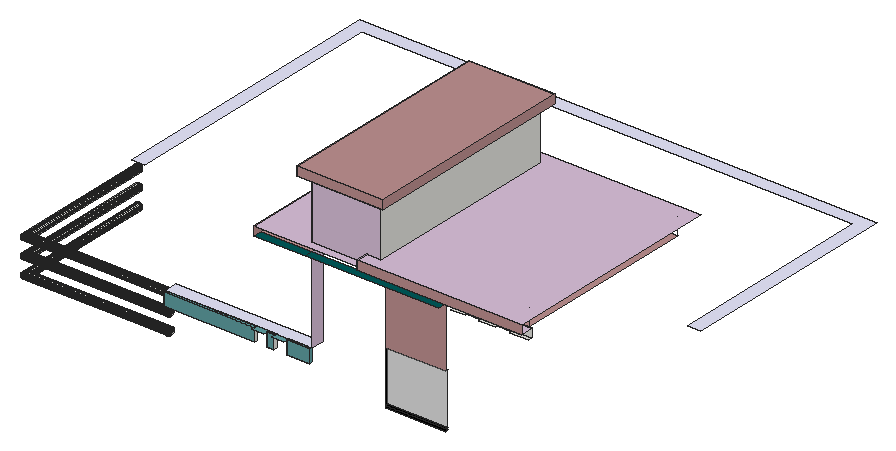
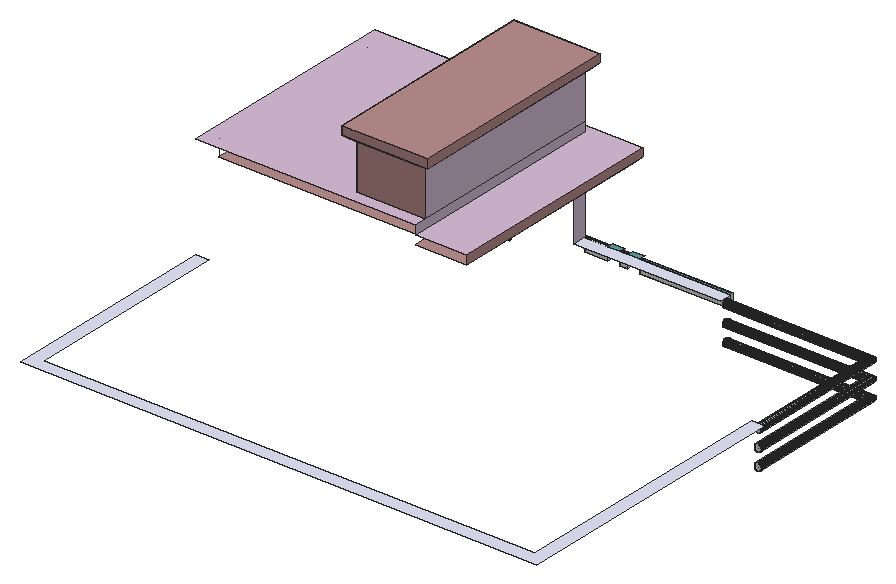
# SketchUp Ruby script. Lengths in inches.
U = 1.inch
M = Sketchup.active_model
def pt(a) = Geom::Point3d.new(a.map { |v| v * U })
def face(e, loops, mat)
  f = e.add_face(loops[0].map { |a| pt(a) })
  loops[1..].each { |l| e.add_face(l.map { |a| pt(a) }).erase! }
  f.material = f.back_material = mat if mat
  f
end
# faces: each face lists its corners as indices into pts; further lists are holes
def faces(e, pts, list, mat = nil) = list.each { |f| face(e, (f[0].is_a?(Array) ? f : [f]).map { |l| l.map { |i| pts[i] } }, mat) }
# xy, xz, yz: faces in a plane at the given z, y or x. An outline is a flat list of corners, or four numbers for a rectangle; further outlines are holes
def ring(l) = l.size == 4 ? [[l[0], l[1]], [l[2], l[1]], [l[2], l[3]], [l[0], l[3]]] : l.each_slice(2).to_a
def flat(e, list, mat, &to3) = list.each { |f| face(e, (f[0].is_a?(Array) ? f : [f]).map { |l| ring(l).map { |u, v| to3.(u, v) } }, mat) }
def xy(e, z, list, mat = nil) = flat(e, list, mat) { |x, y| [x, y, z] }
def xz(e, y, list, mat = nil) = flat(e, list, mat) { |x, z| [x, y, z] }
def yz(e, x, list, mat = nil) = flat(e, list, mat) { |y, z| [x, y, z] }
def lines(e, pts, list) = list.each { |a, b| e.add_line(pt(pts[a]), pt(pts[b])) }
# prism: a flat outline (further loops are holes) pulled along v
def prism(e, loops, v, mat = nil)
  f = face(e, loops, mat); d = Geom::Vector3d.new(v.map { |x| x * U })
  f.pushpull(f.normal.samedirection?(d) ? d.length : -d.length)
end
def box(e, o, s, mat = nil) = prism(e, [[o, [o[0] + s[0], o[1], o[2]], [o[0] + s[0], o[1] + s[1], o[2]], [o[0], o[1] + s[1], o[2]]]], [0, 0, s[2]], mat)
def at(x, y, z, deg = 0) = Geom::Transformation.translation(pt([x, y, z])) * Geom::Transformation.rotation(ORIGIN, Z_AXIS, deg.degrees)
def axes(o, x, y, z) = Geom::Transformation.new([*x, 0, *y, 0, *z, 0, *pt(o).to_a, 1])
def part(name) = M.definitions.add(name)
# library, detail: a bought-in or finely detailed component or shape, given as its bounding box
def library(name, o, s) = part(name).tap { |d| box(d.entities, o, s) }
def detail(e, o, s) = box(e.add_group.entities, o, s)
def put(e, d, t, mat = nil) = e.add_instance(d, t).tap { |i| i.material = mat if mat }
def group(e, t, mat = nil) = e.add_group.tap { |g| g.transformation = t; g.material = mat if mat }.entities
root = M.entities
M.materials.add("[0080_DarkCyan]").color = [0, 89, 89]
M.materials.add("[0081_CadetBlue]").color = [95, 158, 160]
M.materials.add("[0116_Lavender]").color = [230, 230, 250]
M.materials.add("[0118_Thistle]").color = [216, 191, 216]
M.materials.add("[0119_RosyBrown]").color = [188, 143, 143]
M.materials.add("[0137_Black]").color = [0, 0, 0]
M.materials.add("[Translucent Glass Gray]").color = [128, 128, 128]
M.materials["[Translucent Glass Gray]"].alpha = 0.5
xy(root,429,[[528,18,612,21]],"[0137_Black]")
xy(root,432,[[528,18,612,21]],"[0137_Black]")
xy(root,450,[[222,14,348.57,18],[365.51,14,376.32,18],[393.26,14,426,18]],"[0081_CadetBlue]")
xy(root,468,[[348.57,10,365.51,18],[376.32,10,393.26,18],[222,14,348.57,18],[365.51,14,376.32,18],[393.26,14,426,18]],"[0081_CadetBlue]")
xy(root,468,[[222,18,426,36],[12,222,30,222,30,600,714,600,714,312,732,312,732,618,12,618]],"[0116_Lavender]")
xy(root,504,[[528,18,612,21]],"[0137_Black]")
xy(root,588,[[624,12,644.09,12,644.09,15,663.05,15,663.05,12,687.09,12,687.09,15,706.05,15,706.05,12,732,12,732,18,624,18],[389.27,45.6875,387.74,46.01,386.34,46.72,385.18,47.76,384.32,49.07,383.84,50.5625,383.75,52.13,384.07,53.66,384.78,55.06,385.83,56.22,387.14,57.08,388.63,57.57,390.19,57.65,391.72,57.33,393.12,56.62,394.29,55.57,395.14,54.26,395.63,52.77,395.72,51.21,395.39,49.68,394.68,48.28,393.64,47.11,392.33,46.26,390.84,45.77],[389.27,83.6875,387.74,84.01,386.34,84.72,385.18,85.76,384.32,87.07,383.84,88.5625,383.75,90.13,384.07,91.66,384.78,93.06,385.83,94.22,387.14,95.08,388.63,95.57,390.19,95.65,391.72,95.33,393.12,94.62,394.29,93.57,395.14,92.26,395.63,90.77,395.72,89.21,395.39,87.68,394.68,86.28,393.64,85.11,392.33,84.26,390.84,83.77],[389.27,135.125,387.74,135.45,386.34,136.15,385.18,137.2,384.32,138.51,383.84,140,383.75,141.57,384.07,143.1,384.78,144.49,385.83,145.66,387.14,146.52,388.63,147,390.19,147.09,391.72,146.77,393.12,146.06,394.29,145.01,395.14,143.7,395.63,142.21,395.72,140.65,395.39,139.12,394.68,137.72,393.64,136.55,392.33,135.7,390.84,135.21]])
xy(root,588,[[354,6,426,18],[426,6,612,18]],"[0080_DarkCyan]")
xy(root,588,[[[354,18,354,312,426,312,426,294,714,294,714,36,426,36,426,18],[389.27,83.6875,390.84,83.77,392.33,84.26,393.64,85.11,394.68,86.28,395.39,87.68,395.72,89.21,395.63,90.77,395.14,92.26,394.29,93.57,393.12,94.62,391.72,95.33,390.19,95.65,388.63,95.57,387.14,95.08,385.83,94.22,384.78,93.06,384.07,91.66,383.75,90.13,383.84,88.5625,384.32,87.07,385.18,85.76,386.34,84.72,387.74,84.01],[389.27,135.125,390.84,135.21,392.33,135.7,393.64,136.55,394.68,137.72,395.39,139.12,395.72,140.65,395.63,142.21,395.14,143.7,394.29,145.01,393.12,146.06,391.72,146.77,390.19,147.09,388.63,147,387.14,146.52,385.83,145.66,384.78,144.49,384.07,143.1,383.75,141.57,383.84,140,384.32,138.51,385.18,137.2,386.34,136.15,387.74,135.45],[389.27,45.6875,390.84,45.77,392.33,46.26,393.64,47.11,394.68,48.28,395.39,49.68,395.72,51.21,395.63,52.77,395.14,54.26,394.29,55.57,393.12,56.62,391.72,57.33,390.19,57.65,388.63,57.57,387.14,57.08,385.83,56.22,384.78,55.06,384.07,53.66,383.75,52.13,383.84,50.5625,384.32,49.07,385.18,47.76,386.34,46.72,387.74,46.01]]],"[0119_RosyBrown]")
xy(root,600,[[502.63,6,624,18]])
xy(root,600,[[502.63,0,502.63,6,624,6,624,18,732,18,732,0],[354,6,502.63,6,502.63,18,426,18,426,312,354,312]],"[0118_Thistle]")
xy(root,612,[[502.63,0,732,0,732,312,426,312,426,294,522,294,522,18,502.63,18]],"[0118_Thistle]")
xy(root,684,[[426,18,522,294],[426,294,522,306]])
xy(root,684,[[414,6,534,18],[414,18,426,306],[522,18,534,306]],"[0119_RosyBrown]")
xy(root,696,[[414,6,534,306]],"[0119_RosyBrown]")
xz(root,0,[[502.63,600,732,612]],"[0119_RosyBrown]")
xz(root,6,[[414,684,534,696]],"[0119_RosyBrown]")
xz(root,14,[[222,450,348.57,468],[365.51,450,376.32,468],[393.26,450,426,468]],"[0081_CadetBlue]")
xz(root,18,[[222,450,348.57,468],[365.51,450,376.32,468],[393.26,450,426,468],[624,588,732,600]])
xz(root,18,[[426,600,502.63,600,502.63,612,522,612,522,684,426,684]],"[0118_Thistle]")
xz(root,18,[[528,504,612,588]],"[0119_RosyBrown]")
xz(root,18,[[528,429,612,432]],"[0137_Black]")
xz(root,21,[[528,432,612,504]],"[Translucent Glass Gray]")
xz(root,222,[[21.12,407.86,20.59,407.87,20.08,407.94,19.57,408.07,19.07,408.24,18.6,408.47,18.16,408.74,17.74,409.0625,17.36,409.42,17.02,409.82,16.73,410.25,16.48,410.72,16.28,411.2,16.13,411.7,16.04,412.22,16,412.74,16.02,413.26,16.09,413.78,16.21,414.29,16.39,414.78,16.61,415.25,16.89,415.7,17.21,416.11,17.57,416.49,17.97,416.83,18.4,417.125,18.86,417.375,19.34,417.57,19.85,417.72,20.36,417.8125,20.88,417.85,21.41,417.84,21.92,417.77,22.43,417.65,22.93,417.47,23.4,417.24,23.84,416.97,24.26,416.65,24.64,416.29,24.98,415.89,25.27,415.46,25.52,415,25.72,414.51,25.87,414.01,25.96,413.49,26,412.97,25.98,412.45,25.91,411.93,25.79,411.42,25.61,410.93,25.39,410.46,25.11,410.01,24.79,409.6,24.43,409.22,24.03,408.88,23.6,408.58,23.14,408.34,22.66,408.14,22.15,407.99,21.64,407.9],[21.12,431.86,20.59,431.87,20.08,431.94,19.57,432.07,19.07,432.24,18.6,432.47,18.16,432.74,17.74,433.0625,17.36,433.42,17.02,433.82,16.73,434.25,16.48,434.72,16.28,435.2,16.13,435.7,16.04,436.22,16,436.74,16.02,437.26,16.09,437.78,16.21,438.29,16.39,438.78,16.61,439.25,16.89,439.7,17.21,440.11,17.57,440.49,17.97,440.83,18.4,441.125,18.86,441.375,19.34,441.57,19.85,441.72,20.36,441.8125,20.88,441.85,21.41,441.84,21.92,441.77,22.43,441.65,22.93,441.47,23.4,441.24,23.84,440.97,24.26,440.65,24.64,440.29,24.98,439.89,25.27,439.46,25.52,439,25.72,438.51,25.87,438.01,25.96,437.49,26,436.97,25.98,436.45,25.91,435.93,25.79,435.42,25.61,434.93,25.39,434.46,25.11,434.01,24.79,433.6,24.43,433.22,24.03,432.88,23.6,432.58,23.14,432.34,22.66,432.14,22.15,431.99,21.64,431.9],[21.12,455.86,20.59,455.87,20.08,455.94,19.57,456.07,19.07,456.24,18.6,456.47,18.16,456.74,17.74,457.0625,17.36,457.42,17.02,457.82,16.73,458.25,16.48,458.72,16.28,459.2,16.13,459.7,16.04,460.22,16,460.74,16.02,461.26,16.09,461.78,16.21,462.29,16.39,462.78,16.61,463.25,16.89,463.7,17.21,464.11,17.57,464.49,17.97,464.83,18.4,465.125,18.86,465.375,19.34,465.57,19.85,465.72,20.36,465.8125,20.88,465.85,21.41,465.84,21.92,465.77,22.43,465.65,22.93,465.47,23.4,465.24,23.84,464.97,24.26,464.65,24.64,464.29,24.98,463.89,25.27,463.46,25.52,463,25.72,462.51,25.87,462.01,25.96,461.49,26,460.97,25.98,460.45,25.91,459.93,25.79,459.42,25.61,458.93,25.39,458.46,25.11,458.01,24.79,457.6,24.43,457.22,24.03,456.88,23.6,456.58,23.14,456.34,22.66,456.14,22.15,455.99,21.64,455.9]])
xz(root,294,[[426,612,522,684]],"[0119_RosyBrown]")
xz(root,306,[[414,684,534,696]],"[0119_RosyBrown]")
yz(root,222,[[26.48,407.86,25.96,407.95,25.45,408.08,24.97,408.27,24.5,408.51,24.0625,408.79,23.65,409.12,23.28,409.49,22.95,409.9,22.67,410.34,22.43,410.8,22.24,411.29,22.13,411.7,22.11,411.8,22.05,412.14,22.13,411.7,22.28,411.2,22.48,410.72,22.73,410.25,23.02,409.82,23.36,409.42,23.74,409.0625,24.16,408.74,24.6,408.47,25.07,408.24,25.57,408.07,26.08,407.94,26.59,407.87,27.08,407.86],[27.14,407.86,27.64,407.9,28.15,407.99,28.66,408.14,29.14,408.34,29.6,408.58,30.03,408.88,30.43,409.22,30.79,409.6,31.11,410.01,31.39,410.46,31.61,410.93,31.79,411.42,31.91,411.91,31.89,411.8,31.79,411.42,31.76,411.29,31.57,410.8,31.33,410.34,31.05,409.9,30.72,409.49,30.35,409.12,29.9375,408.79,29.5,408.51,29.03,408.27,28.55,408.08,28.04,407.95,27.52,407.86],[31.92,412,31.98,412.4,31.97,412.3125],[22.04,412.24,22.03,412.3125,22.01,412.58],[31.99,412.61,32,412.9,32,412.84],
  [22,412.78,22,412.84,22.01,413.02],[31.98,413.22,31.97,413.4,31.97,413.36],[22.03,413.33,22.03,413.36,22.04,413.45],[31.9,413.82,31.89,413.89,31.89,413.875],[26.48,431.86,25.96,431.95,25.45,432.08,24.97,432.27,24.5,432.51,24.0625,432.79,23.65,433.12,23.28,433.49,22.95,433.9,22.67,434.34,22.43,434.8,22.24,435.29,22.13,435.7,22.11,435.8,22.05,436.14,22.13,435.7,22.28,435.2,22.48,434.72,22.73,434.25,23.02,433.82,23.36,433.42,23.74,433.0625,24.16,432.74,24.6,432.47,25.07,432.24,25.57,432.07,26.08,431.94,26.59,431.87,27.08,431.86],
  [27.14,431.86,27.64,431.9,28.15,431.99,28.66,432.14,29.14,432.34,29.6,432.58,30.03,432.88,30.43,433.22,30.79,433.6,31.11,434.01,31.39,434.46,31.61,434.93,31.79,435.42,31.91,435.91,31.89,435.8,31.79,435.42,31.76,435.29,31.57,434.8,31.33,434.34,31.05,433.9,30.72,433.49,30.35,433.12,29.9375,432.79,29.5,432.51,29.03,432.27,28.55,432.08,28.04,431.95,27.52,431.86],[31.92,436,31.98,436.4,31.97,436.3125],[22.04,436.24,22.03,436.3125,22.01,436.58],[31.99,436.61,32,436.9,32,436.84],[22,436.78,22,436.84,22.01,437.02],
  [31.98,437.22,31.97,437.4,31.97,437.36],[22.03,437.33,22.03,437.36,22.04,437.45],[31.9,437.82,31.89,437.89,31.89,437.875],[14,450,18,468],[26.48,455.86,25.96,455.95,25.45,456.08,24.97,456.27,24.5,456.51,24.0625,456.79,23.65,457.12,23.28,457.49,22.95,457.9,22.67,458.34,22.43,458.8,22.24,459.29,22.13,459.7,22.11,459.8,22.05,460.14,22.13,459.7,22.28,459.2,22.48,458.72,22.73,458.25,23.02,457.82,23.36,457.42,23.74,457.0625,24.16,456.74,24.6,456.47,25.07,456.24,25.57,456.07,26.08,455.94,26.59,455.87,27.08,455.86],
  [27.14,455.86,27.64,455.9,28.15,455.99,28.66,456.14,29.14,456.34,29.6,456.58,30.03,456.88,30.43,457.22,30.79,457.6,31.11,458.01,31.39,458.46,31.61,458.93,31.79,459.42,31.91,459.91,31.89,459.8,31.79,459.42,31.76,459.29,31.57,458.8,31.33,458.34,31.05,457.9,30.72,457.49,30.35,457.12,29.9375,456.79,29.5,456.51,29.03,456.27,28.55,456.08,28.04,455.95,27.52,455.86],[31.92,460,31.98,460.4,31.97,460.3125],[22.04,460.24,22.03,460.3125,22.01,460.58],[31.99,460.61,32,460.9,32,460.84],[22,460.78,22,460.84,22.01,461.02],
  [31.98,461.22,31.97,461.4,31.97,461.36],[22.03,461.33,22.03,461.36,22.04,461.45],[31.9,461.82,31.89,461.89,31.89,461.875]])
yz(root,348.57,[[14,450,18,468]])
yz(root,354,[[6,588,312,600]],"[0119_RosyBrown]")
yz(root,365.51,[[14,450,18,468]])
yz(root,376.32,[[14,450,18,468]])
yz(root,393.26,[[14,450,18,468]])
yz(root,414,[[6,684,306,696]],"[0119_RosyBrown]")
yz(root,426,[[14,450,18,468]],"[0081_CadetBlue]")
yz(root,426,[[18,468,36,588],[18,600,312,612],[18,612,294,684]],"[0118_Thistle]")
yz(root,502.63,[[0,600,18,612]],"[0118_Thistle]")
yz(root,522,[[18,612,294,684]])
yz(root,528,[[18,432,21,504]],"[0137_Black]")
yz(root,534,[[6,684,306,696]],"[0119_RosyBrown]")
p = [[19.57,222,408.07],[20.08,222,407.94],[20.08,26.08,407.94],[19.57,25.57,408.07],[222,26.08,407.94],[222,25.57,408.07],
  [20.59,222,407.87],[20.59,26.59,407.87],[222,26.59,407.87],[21.12,222,407.86],[21.12,27.12,407.86],[222,27.12,407.86],
  [222,27.08,407.86],[21.64,222,407.9],[21.64,27.64,407.9],[222,27.64,407.9],[222,27.14,407.86],[22.15,222,407.99],
  [22.15,28.15,407.99],[222,28.15,407.99],[22.66,222,408.14],[22.66,28.66,408.14],[222,28.66,408.14],[19.07,222,408.24],
  [19.07,25.07,408.24],[222,25.07,408.24],[23.14,222,408.34],[23.14,29.14,408.34],[222,29.14,408.34],[18.6,222,408.47],
  [18.6,24.6,408.47],[222,24.6,408.47],[23.6,222,408.58],[23.6,29.6,408.58],[222,29.6,408.58],[18.16,222,408.74],
  [18.16,24.16,408.74],[222,24.16,408.74],[24.03,222,408.88],[24.03,30.03,408.88],[222,30.03,408.88],[17.74,222,409.0625],
  [17.74,23.74,409.0625],[222,23.74,409.0625],[24.43,222,409.22],[24.43,30.43,409.22],[222,30.43,409.22],[17.36,222,409.42],
  [17.36,23.36,409.42],[222,23.36,409.42],[24.79,222,409.6],[24.79,30.79,409.6],[222,30.79,409.6],[17.02,222,409.82],
  [17.02,23.02,409.82],[222,23.02,409.82],[25.11,222,410.01],[25.11,31.11,410.01],[222,31.11,410.01],[16.73,222,410.25],
  [16.73,22.73,410.25],[222,22.73,410.25],[25.39,222,410.46],[25.39,31.39,410.46],[222,31.39,410.46],[16.48,222,410.72],
  [16.48,22.48,410.72],[222,22.48,410.72],[25.61,222,410.93],[25.61,31.61,410.93],[222,31.61,410.93],[16.28,222,411.2],
  [16.28,22.28,411.2],[222,22.28,411.2],[25.79,222,411.42],[25.79,31.79,411.42],[222,31.79,411.42],[16.13,222,411.7],
  [16.13,22.13,411.7],[222,22.13,411.7],[25.91,222,411.93],[25.91,31.91,411.93],[222,31.91,411.93],[222,31.91,411.91],
  [16.04,222,412.22],[16.04,22.04,412.22],[222,22.05,412.14],[222,22.04,412.22],[25.98,222,412.45],[25.98,31.98,412.45],
  [222,31.98,412.45],[222,31.98,412.4],[222,31.92,412],[16,222,412.74],[16,22,412.74],[222,22.04,412.24],
  [222,22.01,412.58],[222,22,412.74],[26,222,412.97],[26,32,412.97],[222,32,412.97],[222,32,412.9],
  [222,31.99,412.61],[16.02,222,413.26],[16.02,22.02,413.26],[222,22,412.78],[222,22.01,413.02],[222,22.02,413.26],
  [25.96,222,413.49],[25.96,31.96,413.49],[222,31.96,413.49],[222,31.97,413.4],[222,31.98,413.22],[16.09,222,413.78],
  [16.09,22.09,413.78],[222,22.03,413.33],[222,22.04,413.45],[222,22.09,413.78],[25.87,222,414.01],[25.87,31.87,414.01],
  [222,31.87,414.01],[222,31.89,413.89],[222,31.9,413.82],[16.21,222,414.29],[16.21,22.21,414.29],[222,22.11,413.87],
  [222,22.11,413.875],[222,22.11,413.88],[222,22.21,414.29],[25.72,222,414.51],[25.72,31.72,414.51],[222,31.72,414.51],
  [222,31.76,414.38],[16.39,222,414.78],[16.39,22.39,414.78],[222,22.39,414.78],[25.52,222,415],[25.52,31.52,415],
  [222,31.52,415],[16.61,222,415.25],[16.61,22.61,415.25],[222,22.61,415.25],[25.27,222,415.46],[25.27,31.27,415.46],
  [222,31.27,415.46],[16.89,222,415.7],[16.89,22.89,415.7],[222,22.89,415.7],[24.98,222,415.89],[24.98,30.98,415.89],
  [222,30.98,415.89],[17.21,222,416.11],[17.21,23.21,416.11],[222,23.21,416.11],[24.64,222,416.29],[24.64,30.64,416.29],
  [222,30.64,416.29],[17.57,222,416.49],[17.57,23.57,416.49],[222,23.57,416.49],[24.26,222,416.65],[24.26,30.26,416.65],
  [222,30.26,416.65],[17.97,222,416.83],[17.97,23.97,416.83],[222,23.97,416.83],[23.84,222,416.97],[23.84,29.84,416.97],
  [222,29.84,416.97],[18.4,222,417.125],[18.4,24.4,417.125],[222,24.4,417.125],[23.4,222,417.24],[23.4,29.4,417.24],
  [222,29.4,417.24],[18.86,222,417.375],[18.86,24.86,417.375],[222,24.86,417.375],[22.93,222,417.47],[22.93,28.93,417.47],
  [222,28.93,417.47],[19.34,222,417.57],[19.34,25.34,417.57],[222,25.34,417.57],[22.43,222,417.65],[22.43,28.43,417.65],
  [222,28.43,417.65],[19.85,222,417.72],[19.85,25.85,417.72],[222,25.85,417.72],[21.92,222,417.77],[21.92,27.92,417.77],
  [222,27.92,417.77],[20.36,222,417.8125],[20.36,26.36,417.8125],[222,26.36,417.8125],[20.88,222,417.85],[20.88,26.88,417.85],
  [222,26.88,417.85],[21.41,222,417.84],[21.41,27.41,417.84],[222,27.41,417.84],[19.57,222,432.07],[20.08,222,431.94],
  [20.08,26.08,431.94],[19.57,25.57,432.07],[222,26.08,431.94],[222,25.57,432.07],[20.59,222,431.87],[20.59,26.59,431.87],
  [222,26.59,431.87],[21.12,222,431.86],[21.12,27.12,431.86],[222,27.12,431.86],[222,27.08,431.86],[21.64,222,431.9],
  [21.64,27.64,431.9],[222,27.64,431.9],[222,27.14,431.86],[22.15,222,431.99],[22.15,28.15,431.99],[222,28.15,431.99],
  [22.66,222,432.14],[22.66,28.66,432.14],[222,28.66,432.14],[19.07,222,432.24],[19.07,25.07,432.24],[222,25.07,432.24],
  [23.14,222,432.34],[23.14,29.14,432.34],[222,29.14,432.34],[18.6,222,432.47],[18.6,24.6,432.47],[222,24.6,432.47],
  [23.6,222,432.58],[23.6,29.6,432.58],[222,29.6,432.58],[18.16,222,432.74],[18.16,24.16,432.74],[222,24.16,432.74],
  [24.03,222,432.88],[24.03,30.03,432.88],[222,30.03,432.88],[17.74,222,433.0625],[17.74,23.74,433.0625],[222,23.74,433.0625],
  [24.43,222,433.22],[24.43,30.43,433.22],[222,30.43,433.22],[17.36,222,433.42],[17.36,23.36,433.42],[222,23.36,433.42],
  [24.79,222,433.6],[24.79,30.79,433.6],[222,30.79,433.6],[17.02,222,433.82],[17.02,23.02,433.82],[222,23.02,433.82],
  [25.11,222,434.01],[25.11,31.11,434.01],[222,31.11,434.01],[16.73,222,434.25],[16.73,22.73,434.25],[222,22.73,434.25],
  [25.39,222,434.46],[25.39,31.39,434.46],[222,31.39,434.46],[16.48,222,434.72],[16.48,22.48,434.72],[222,22.48,434.72],
  [25.61,222,434.93],[25.61,31.61,434.93],[222,31.61,434.93],[16.28,222,435.2],[16.28,22.28,435.2],[222,22.28,435.2],
  [25.79,222,435.42],[25.79,31.79,435.42],[222,31.79,435.42],[16.13,222,435.7],[16.13,22.13,435.7],[222,22.13,435.7],
  [25.91,222,435.93],[25.91,31.91,435.93],[222,31.91,435.93],[222,31.91,435.91],[16.04,222,436.22],[16.04,22.04,436.22],
  [222,22.05,436.14],[222,22.04,436.22],[25.98,222,436.45],[25.98,31.98,436.45],[222,31.98,436.45],[222,31.98,436.4],
  [222,31.92,436],[16,222,436.74],[16,22,436.74],[222,22.04,436.24],[222,22.01,436.58],[222,22,436.74],
  [26,222,436.97],[26,32,436.97],[222,32,436.97],[222,32,436.9],[222,31.99,436.61],[16.02,222,437.26],
  [16.02,22.02,437.26],[222,22,436.78],[222,22.01,437.02],[222,22.02,437.26],[25.96,222,437.49],[25.96,31.96,437.49],
  [222,31.96,437.49],[222,31.97,437.4],[222,31.98,437.22],[16.09,222,437.78],[16.09,22.09,437.78],[222,22.03,437.33],
  [222,22.04,437.45],[222,22.09,437.78],[25.87,222,438.01],[25.87,31.87,438.01],[222,31.87,438.01],[222,31.89,437.89],
  [222,31.9,437.82],[16.21,222,438.29],[16.21,22.21,438.29],[222,22.11,437.87],[222,22.11,437.875],[222,22.11,437.88],
  [222,22.21,438.29],[25.72,222,438.51],[25.72,31.72,438.51],[222,31.72,438.51],[222,31.76,438.38],[16.39,222,438.78],
  [16.39,22.39,438.78],[222,22.39,438.78],[25.52,222,439],[25.52,31.52,439],[222,31.52,439],[16.61,222,439.25],
  [16.61,22.61,439.25],[222,22.61,439.25],[25.27,222,439.46],[25.27,31.27,439.46],[222,31.27,439.46],[16.89,222,439.7],
  [16.89,22.89,439.7],[222,22.89,439.7],[24.98,222,439.89],[24.98,30.98,439.89],[222,30.98,439.89],[17.21,222,440.11],
  [17.21,23.21,440.11],[222,23.21,440.11],[24.64,222,440.29],[24.64,30.64,440.29],[222,30.64,440.29],[17.57,222,440.49],
  [17.57,23.57,440.49],[222,23.57,440.49],[24.26,222,440.65],[24.26,30.26,440.65],[222,30.26,440.65],[17.97,222,440.83],
  [17.97,23.97,440.83],[222,23.97,440.83],[23.84,222,440.97],[23.84,29.84,440.97],[222,29.84,440.97],[18.4,222,441.125],
  [18.4,24.4,441.125],[222,24.4,441.125],[23.4,222,441.24],[23.4,29.4,441.24],[222,29.4,441.24],[18.86,222,441.375],
  [18.86,24.86,441.375],[222,24.86,441.375],[22.93,222,441.47],[22.93,28.93,441.47],[222,28.93,441.47],[19.34,222,441.57],
  [19.34,25.34,441.57],[222,25.34,441.57],[22.43,222,441.65],[22.43,28.43,441.65],[222,28.43,441.65],[19.85,222,441.72],
  [19.85,25.85,441.72],[222,25.85,441.72],[21.92,222,441.77],[21.92,27.92,441.77],[222,27.92,441.77],[20.36,222,441.8125],
  [20.36,26.36,441.8125],[222,26.36,441.8125],[20.88,222,441.85],[20.88,26.88,441.85],[222,26.88,441.85],[21.41,222,441.84],
  [21.41,27.41,441.84],[222,27.41,441.84],[19.57,222,456.07],[20.08,222,455.94],[20.08,26.08,455.94],[19.57,25.57,456.07],
  [222,26.08,455.94],[222,25.57,456.07],[20.59,222,455.87],[20.59,26.59,455.87],[222,26.59,455.87],[21.12,222,455.86],
  [21.12,27.12,455.86],[222,27.12,455.86],[222,27.08,455.86],[21.64,222,455.9],[21.64,27.64,455.9],[222,27.64,455.9],
  [222,27.14,455.86],[22.15,222,455.99],[22.15,28.15,455.99],[222,28.15,455.99],[22.66,222,456.14],[22.66,28.66,456.14],
  [222,28.66,456.14],[19.07,222,456.24],[19.07,25.07,456.24],[222,25.07,456.24],[23.14,222,456.34],[23.14,29.14,456.34],
  [222,29.14,456.34],[18.6,222,456.47],[18.6,24.6,456.47],[222,24.6,456.47],[23.6,222,456.58],[23.6,29.6,456.58],
  [222,29.6,456.58],[18.16,222,456.74],[18.16,24.16,456.74],[222,24.16,456.74],[24.03,222,456.88],[24.03,30.03,456.88],
  [222,30.03,456.88],[17.74,222,457.0625],[17.74,23.74,457.0625],[222,23.74,457.0625],[24.43,222,457.22],[24.43,30.43,457.22],
  [222,30.43,457.22],[17.36,222,457.42],[17.36,23.36,457.42],[222,23.36,457.42],[24.79,222,457.6],[24.79,30.79,457.6],
  [222,30.79,457.6],[17.02,222,457.82],[17.02,23.02,457.82],[222,23.02,457.82],[25.11,222,458.01],[25.11,31.11,458.01],
  [222,31.11,458.01],[16.73,222,458.25],[16.73,22.73,458.25],[222,22.73,458.25],[25.39,222,458.46],[25.39,31.39,458.46],
  [222,31.39,458.46],[16.48,222,458.72],[16.48,22.48,458.72],[222,22.48,458.72],[25.61,222,458.93],[25.61,31.61,458.93],
  [222,31.61,458.93],[16.28,222,459.2],[16.28,22.28,459.2],[222,22.28,459.2],[25.79,222,459.42],[25.79,31.79,459.42],
  [222,31.79,459.42],[16.13,222,459.7],[16.13,22.13,459.7],[222,22.13,459.7],[25.91,222,459.93],[25.91,31.91,459.93],
  [222,31.91,459.93],[222,31.91,459.91],[16.04,222,460.22],[16.04,22.04,460.22],[222,22.05,460.14],[222,22.04,460.22],
  [25.98,222,460.45],[25.98,31.98,460.45],[222,31.98,460.45],[222,31.98,460.4],[222,31.92,460],[16,222,460.74],
  [16,22,460.74],[222,22.04,460.24],[222,22.01,460.58],[222,22,460.74],[26,222,460.97],[26,32,460.97],
  [222,32,460.97],[222,32,460.9],[222,31.99,460.61],[16.02,222,461.26],[16.02,22.02,461.26],[222,22,460.78],
  [222,22.01,461.02],[222,22.02,461.26],[25.96,222,461.49],[25.96,31.96,461.49],[222,31.96,461.49],[222,31.97,461.4],
  [222,31.98,461.22],[16.09,222,461.78],[16.09,22.09,461.78],[222,22.03,461.33],[222,22.04,461.45],[222,22.09,461.78],
  [25.87,222,462.01],[25.87,31.87,462.01],[222,31.87,462.01],[222,31.89,461.89],[222,31.9,461.82],[16.21,222,462.29],
  [16.21,22.21,462.29],[222,22.11,461.87],[222,22.11,461.875],[222,22.11,461.88],[222,22.21,462.29],[25.72,222,462.51],
  [25.72,31.72,462.51],[222,31.72,462.51],[222,31.76,462.38],[16.39,222,462.78],[16.39,22.39,462.78],[222,22.39,462.78],
  [25.52,222,463],[25.52,31.52,463],[222,31.52,463],[16.61,222,463.25],[16.61,22.61,463.25],[222,22.61,463.25],
  [25.27,222,463.46],[25.27,31.27,463.46],[222,31.27,463.46],[16.89,222,463.7],[16.89,22.89,463.7],[222,22.89,463.7],
  [24.98,222,463.89],[24.98,30.98,463.89],[222,30.98,463.89],[17.21,222,464.11],[17.21,23.21,464.11],[222,23.21,464.11],
  [24.64,222,464.29],[24.64,30.64,464.29],[222,30.64,464.29],[17.57,222,464.49],[17.57,23.57,464.49],[222,23.57,464.49],
  [24.26,222,464.65],[24.26,30.26,464.65],[222,30.26,464.65],[17.97,222,464.83],[17.97,23.97,464.83],[222,23.97,464.83],
  [23.84,222,464.97],[23.84,29.84,464.97],[222,29.84,464.97],[18.4,222,465.125],[18.4,24.4,465.125],[222,24.4,465.125],
  [23.4,222,465.24],[23.4,29.4,465.24],[222,29.4,465.24],[18.86,222,465.375],[18.86,24.86,465.375],[222,24.86,465.375],
  [22.93,222,465.47],[22.93,28.93,465.47],[222,28.93,465.47],[19.34,222,465.57],[19.34,25.34,465.57],[222,25.34,465.57],
  [22.43,222,465.65],[22.43,28.43,465.65],[222,28.43,465.65],[19.85,222,465.72],[19.85,25.85,465.72],[222,25.85,465.72],
  [21.92,222,465.77],[21.92,27.92,465.77],[222,27.92,465.77],[20.36,222,465.8125],[20.36,26.36,465.8125],[222,26.36,465.8125],
  [20.88,222,465.85],[20.88,26.88,465.85],[222,26.88,465.85],[21.41,222,465.84],[21.41,27.41,465.84],[222,27.41,465.84],
  [714,294,588],[714,294,612],[714,36,588],[714,36,612],[21,222,412.86],[21,27,412.86],
  [222,27,412.86],[21,222,436.86],[21,27,436.86],[222,27,436.86],[21,222,460.86],[21,27,460.86],
  [222,27,460.86]]
faces(root,p,[[0,1,2,3],[3,2,4,5],[1,6,7,2],[2,7,8,4],[6,9,10,7],[7,10,11,12,8],[9,13,14,10],[10,14,15,16,11],
  [13,17,18,14],[14,18,19,15],[17,20,21,18],[18,21,22,19],[23,0,3,24],[24,3,5,25],[20,26,27,21],[21,27,28,22],
  [29,23,24,30],[30,24,25,31],[26,32,33,27],[27,33,34,28],[35,29,30,36],[36,30,31,37],[32,38,39,33],[33,39,40,34],
  [41,35,36,42],[42,36,37,43],[38,44,45,39],[39,45,46,40],[47,41,42,48],[48,42,43,49],[44,50,51,45],[45,51,52,46],
  [53,47,48,54],[54,48,49,55],[50,56,57,51],[51,57,58,52],[59,53,54,60],[60,54,55,61],[56,62,63,57],[57,63,64,58],
  [65,59,60,66],[66,60,61,67],[62,68,69,63],[63,69,70,64],[71,65,66,72],[72,66,67,73],[68,74,75,69],[69,75,76,70],
  [77,71,72,78],[78,72,73,79],[74,80,81,75],[75,81,82,83,76],[84,77,78,85],[85,78,79,86,87],[80,88,89,81],[81,89,90,91,92,82],
  [93,84,85,94],[94,85,87,95,96,97],[88,98,99,89],[89,99,100,101,102,90],[103,93,94,104],[104,94,97,105,106,107],[98,108,109,99],[99,109,110,111,112,100],
  [113,103,104,114],[114,104,107,115,116,117],[108,118,119,109],[109,119,120,121,122,110],[123,113,114,124],[124,114,117,125,126,127,128],[118,129,130,119],[119,130,131,132,120],
  [133,123,124,134],[134,124,128,135],[129,136,137,130],[130,137,138,131],[139,133,134,140],[140,134,135,141],[136,142,143,137],[137,143,144,138],
  [145,139,140,146],[146,140,141,147],[142,148,149,143],[143,149,150,144],[151,145,146,152],[152,146,147,153],[148,154,155,149],[149,155,156,150],
  [157,151,152,158],[158,152,153,159],[154,160,161,155],[155,161,162,156],[163,157,158,164],[164,158,159,165],[160,166,167,161],[161,167,168,162],
  [169,163,164,170],[170,164,165,171],[166,172,173,167],[167,173,174,168],[175,169,170,176],[176,170,171,177],[172,178,179,173],[173,179,180,174],
  [181,175,176,182],[182,176,177,183],[178,184,185,179],[179,185,186,180],[187,181,182,188],[188,182,183,189],[184,190,191,185],[185,191,192,186],
  [193,187,188,194],[194,188,189,195],[196,193,194,197],[197,194,195,198],[199,196,197,200],[200,197,198,201],[190,199,200,191],[191,200,201,192],
  [202,203,204,205],[205,204,206,207],[203,208,209,204],[204,209,210,206],[208,211,212,209],[209,212,213,214,210],[211,215,216,212],[212,216,217,218,213],
  [215,219,220,216],[216,220,221,217],[219,222,223,220],[220,223,224,221],[225,202,205,226],[226,205,207,227],[222,228,229,223],[223,229,230,224],
  [231,225,226,232],[232,226,227,233],[228,234,235,229],[229,235,236,230],[237,231,232,238],[238,232,233,239],[234,240,241,235],[235,241,242,236],
  [243,237,238,244],[244,238,239,245],[240,246,247,241],[241,247,248,242],[249,243,244,250],[250,244,245,251],[246,252,253,247],[247,253,254,248],
  [255,249,250,256],[256,250,251,257],[252,258,259,253],[253,259,260,254],[261,255,256,262],[262,256,257,263],[258,264,265,259],[259,265,266,260],
  [267,261,262,268],[268,262,263,269],[264,270,271,265],[265,271,272,266],[273,267,268,274],[274,268,269,275],[270,276,277,271],[271,277,278,272],
  [279,273,274,280],[280,274,275,281],[276,282,283,277],[277,283,284,285,278],[286,279,280,287],[287,280,281,288,289],[282,290,291,283],[283,291,292,293,294,284],
  [295,286,287,296],[296,287,289,297,298,299],[290,300,301,291],[291,301,302,303,304,292],[305,295,296,306],[306,296,299,307,308,309],[300,310,311,301],[301,311,312,313,314,302],
  [315,305,306,316],[316,306,309,317,318,319],[310,320,321,311],[311,321,322,323,324,312],[325,315,316,326],[326,316,319,327,328,329,330],[320,331,332,321],[321,332,333,334,322],
  [335,325,326,336],[336,326,330,337],[331,338,339,332],[332,339,340,333],[341,335,336,342],[342,336,337,343],[338,344,345,339],[339,345,346,340],
  [347,341,342,348],[348,342,343,349],[344,350,351,345],[345,351,352,346],[353,347,348,354],[354,348,349,355],[350,356,357,351],[351,357,358,352],
  [359,353,354,360],[360,354,355,361],[356,362,363,357],[357,363,364,358],[365,359,360,366],[366,360,361,367],[362,368,369,363],[363,369,370,364],
  [371,365,366,372],[372,366,367,373],[368,374,375,369],[369,375,376,370],[377,371,372,378],[378,372,373,379],[374,380,381,375],[375,381,382,376],
  [383,377,378,384],[384,378,379,385],[380,386,387,381],[381,387,388,382],[389,383,384,390],[390,384,385,391],[386,392,393,387],[387,393,394,388],
  [395,389,390,396],[396,390,391,397],[398,395,396,399],[399,396,397,400],[401,398,399,402],[402,399,400,403],[392,401,402,393],[393,402,403,394],
  [404,405,406,407],[407,406,408,409],[405,410,411,406],[406,411,412,408],[410,413,414,411],[411,414,415,416,412],[413,417,418,414],[414,418,419,420,415],
  [417,421,422,418],[418,422,423,419],[421,424,425,422],[422,425,426,423],[427,404,407,428],[428,407,409,429],[424,430,431,425],[425,431,432,426],
  [433,427,428,434],[434,428,429,435],[430,436,437,431],[431,437,438,432],[439,433,434,440],[440,434,435,441],[436,442,443,437],[437,443,444,438],
  [445,439,440,446],[446,440,441,447],[442,448,449,443],[443,449,450,444],[451,445,446,452],[452,446,447,453],[448,454,455,449],[449,455,456,450],
  [457,451,452,458],[458,452,453,459],[454,460,461,455],[455,461,462,456],[463,457,458,464],[464,458,459,465],[460,466,467,461],[461,467,468,462],
  [469,463,464,470],[470,464,465,471],[466,472,473,467],[467,473,474,468],[475,469,470,476],[476,470,471,477],[472,478,479,473],[473,479,480,474],
  [481,475,476,482],[482,476,477,483],[478,484,485,479],[479,485,486,487,480],[488,481,482,489],[489,482,483,490,491],[484,492,493,485],[485,493,494,495,496,486],
  [497,488,489,498],[498,489,491,499,500,501],[492,502,503,493],[493,503,504,505,506,494],[507,497,498,508],[508,498,501,509,510,511],[502,512,513,503],[503,513,514,515,516,504],
  [517,507,508,518],[518,508,511,519,520,521],[512,522,523,513],[513,523,524,525,526,514],[527,517,518,528],[528,518,521,529,530,531,532],[522,533,534,523],[523,534,535,536,524],
  [537,527,528,538],[538,528,532,539],[533,540,541,534],[534,541,542,535],[543,537,538,544],[544,538,539,545],[540,546,547,541],[541,547,548,542],
  [549,543,544,550],[550,544,545,551],[546,552,553,547],[547,553,554,548],[555,549,550,556],[556,550,551,557],[552,558,559,553],[553,559,560,554],
  [561,555,556,562],[562,556,557,563],[558,564,565,559],[559,565,566,560],[567,561,562,568],[568,562,563,569],[564,570,571,565],[565,571,572,566],
  [573,567,568,574],[574,568,569,575],[570,576,577,571],[571,577,578,572],[579,573,574,580],[580,574,575,581],[576,582,583,577],[577,583,584,578],
  [585,579,580,586],[586,580,581,587],[582,588,589,583],[583,589,590,584],[591,585,586,592],[592,586,587,593],[588,594,595,589],[589,595,596,590],
  [597,591,592,598],[598,592,593,599],[600,597,598,601],[601,598,599,602],[603,600,601,604],[604,601,602,605],[594,603,604,595],[595,604,605,596]])
lines(root,p,[[606,607],[608,609],[610,611],[611,612],[613,614],[614,615],[616,617],[617,618]])
